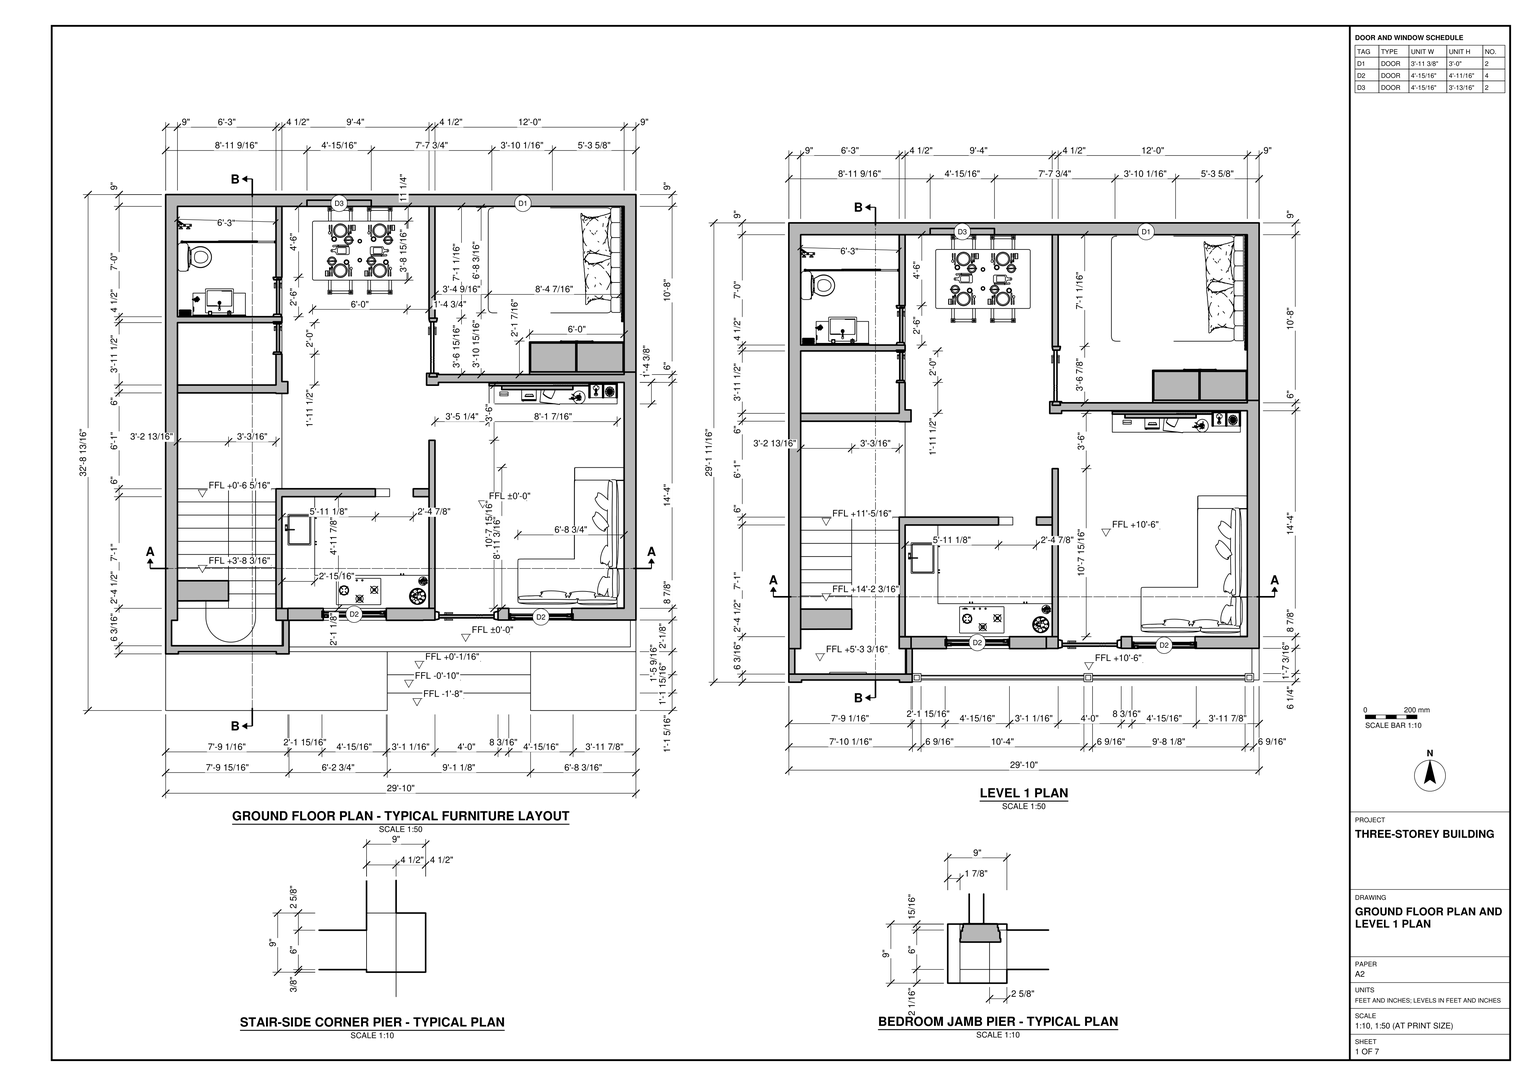
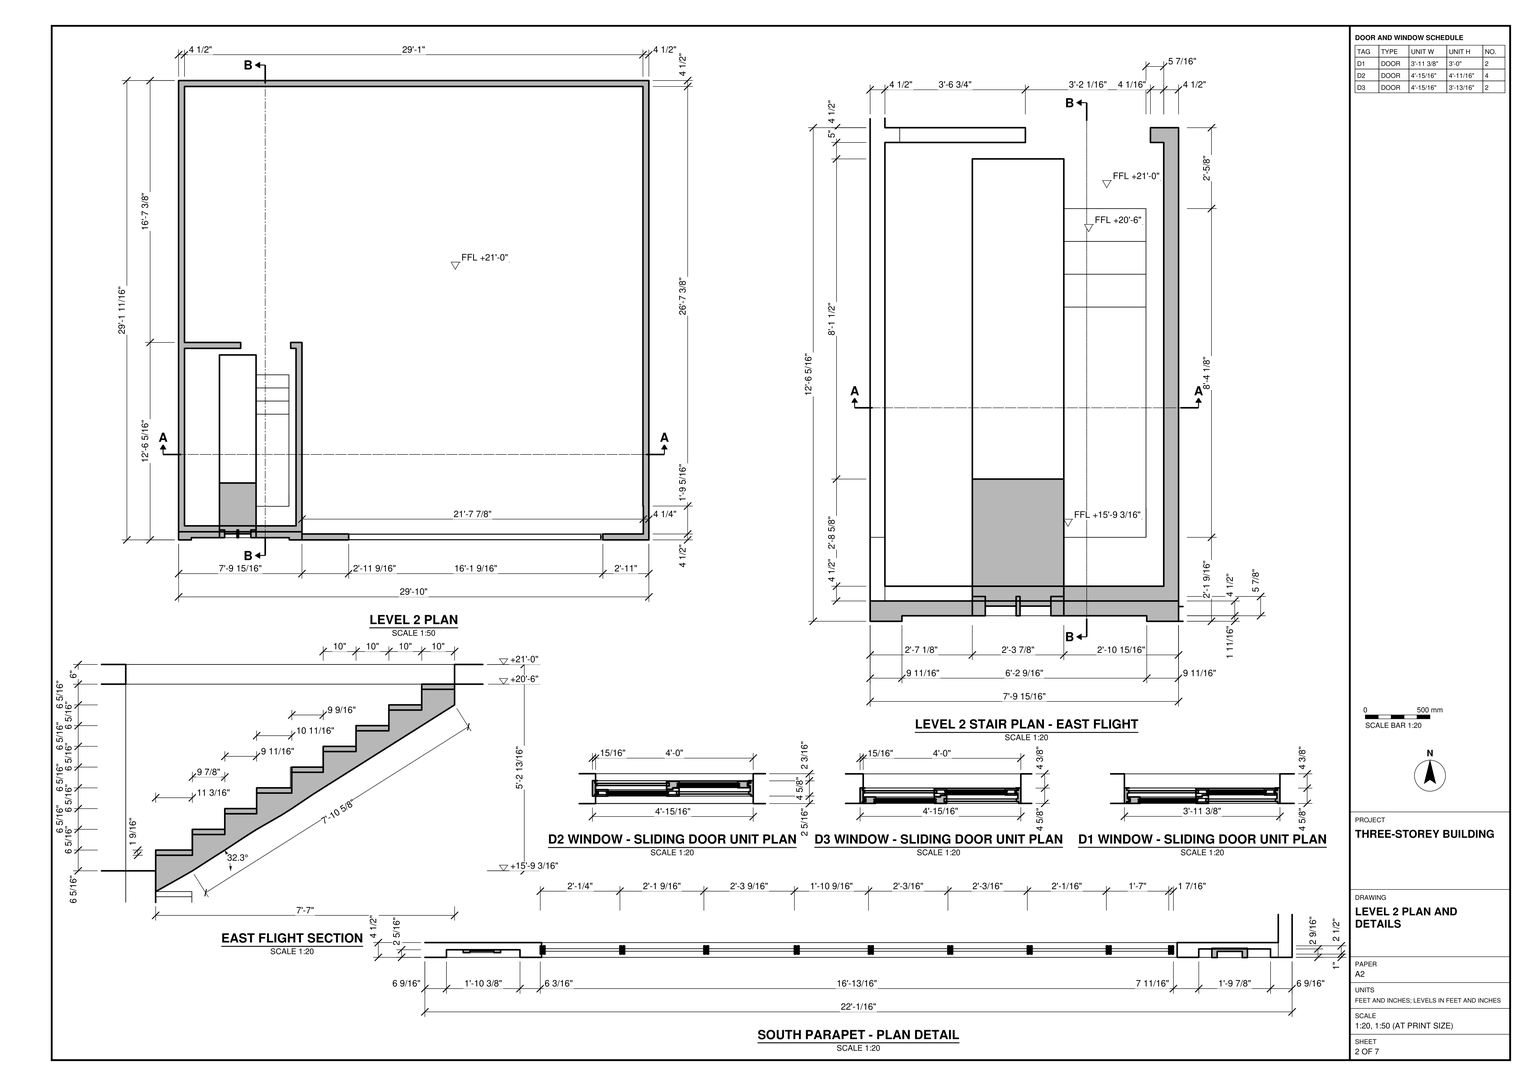
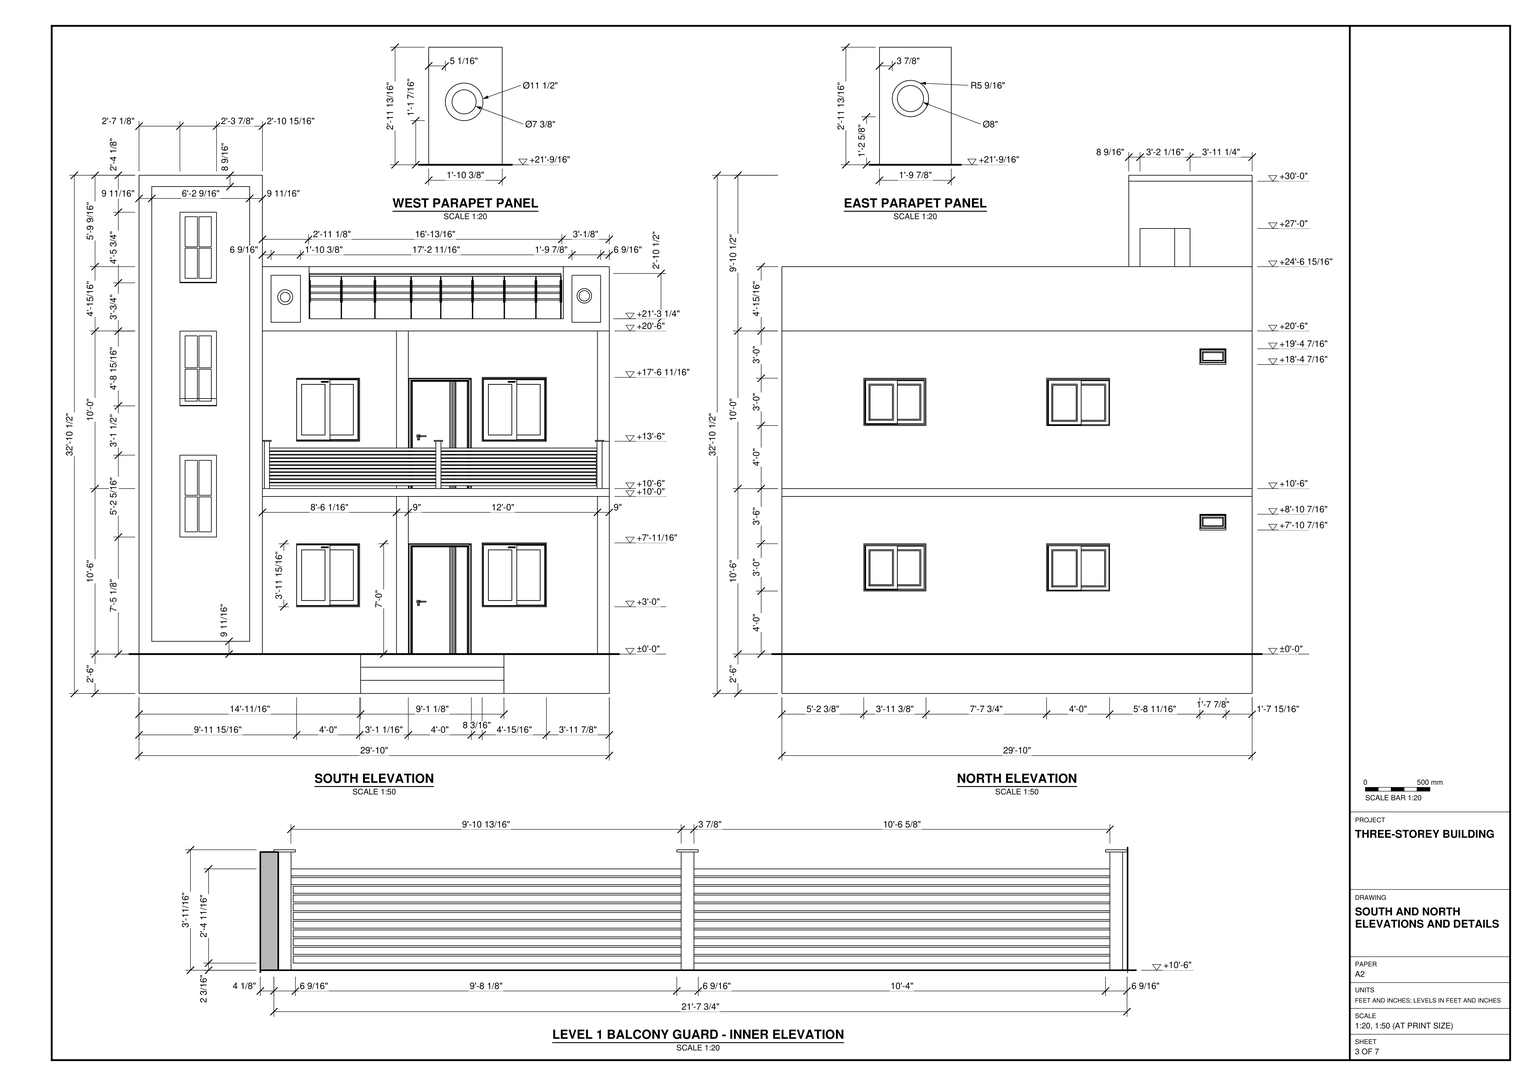
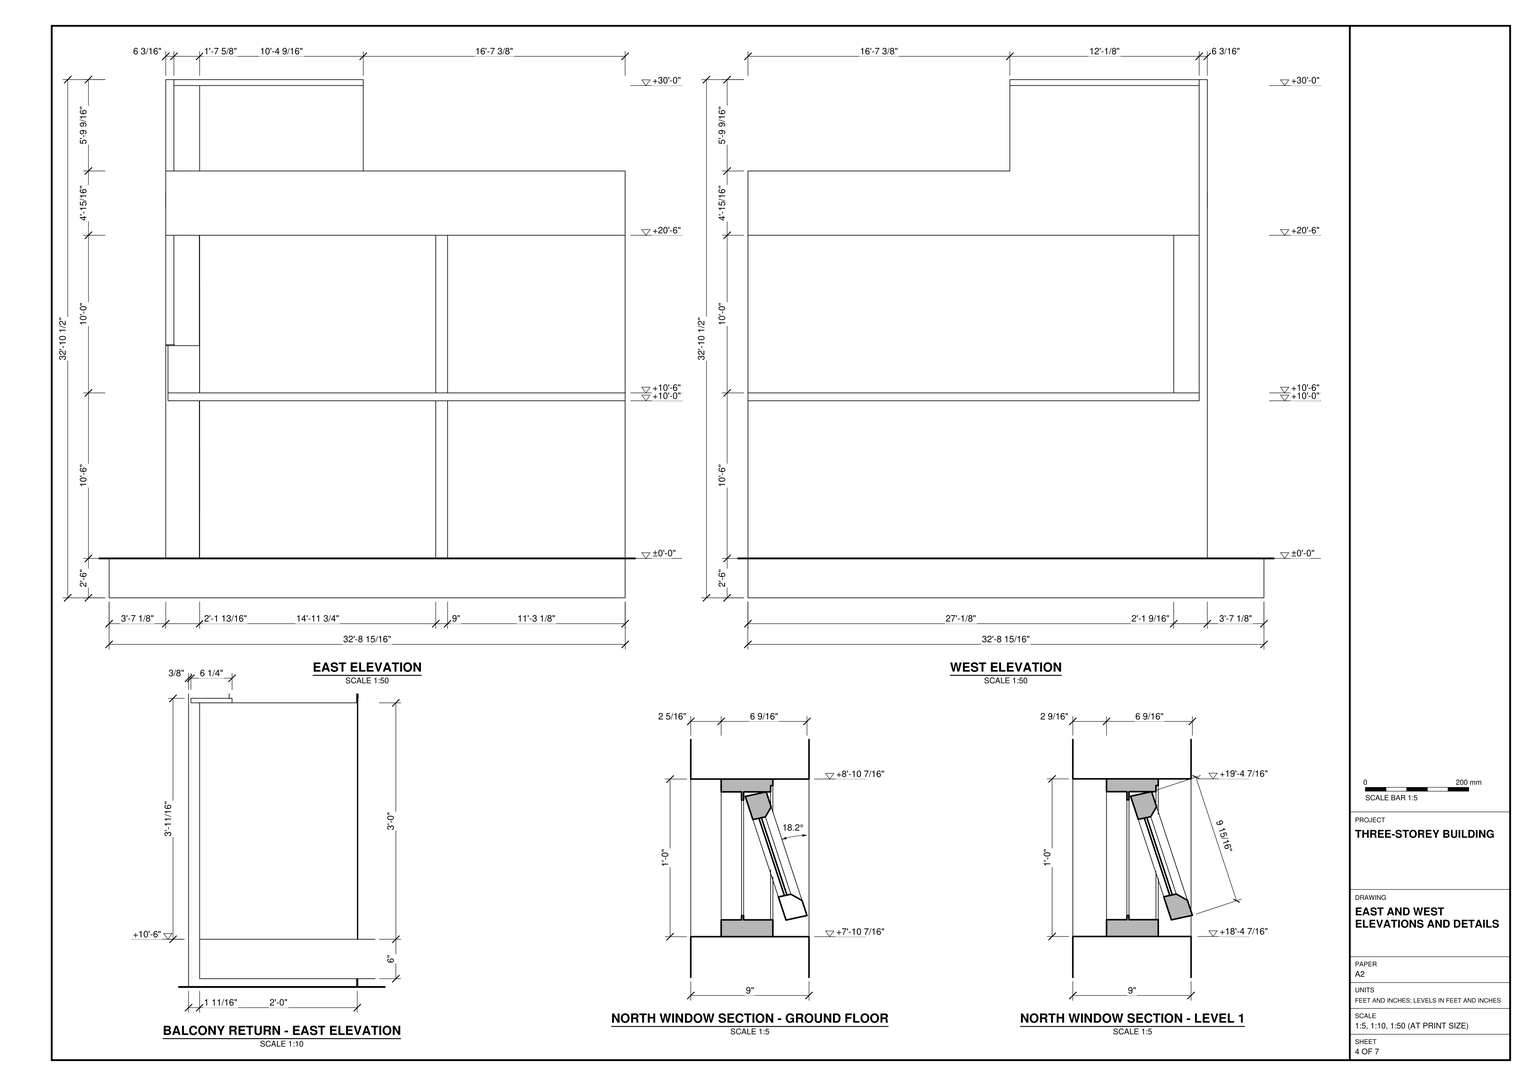
Build the residential building in SketchUp from task_files/diagram_01.pdf. Work in feet and inches. Orient the entrance toward the south and set the overall extents to 29'-10" east to west, 32'-8 15/16" north to south and 32'-10 1/2" from the base to the highest point. Use storey reference levels of ±0'-0", +10'-6" and +20'-6". Distinguish the upper reference level from the terrace surface at +21'-0".

Follow the ground-floor and Level 1 plans for the walls, piers, doorways and window openings. Use the wall thicknesses dimensioned at each location. On both furnished floors, place the stair at the southwest, the bathroom at the northwest, the dining area between the bathroom and bedroom, and the living area at the southeast. Fit the kitchen counters, sink and cooktop, and match the plan footprints and orientations of the dining table and chairs, bed, bedroom storage and corner sofa.

Model the base, entrance steps, floor slabs, stair flights and landings. Use the sections to carry the stair through to its enclosure above the flat roof terrace. Match the south elevation's stacked stair windows, Level 1 balcony guard and roof parapet with its rail opening and end panels.

Keep the walls, slabs and roof as separate groups or components, group each furniture or joinery piece separately, and use components for repeated parts. Decor and loose items may be any suitable library components. Save one SketchUp model as output_files/three_storey_residential_building_with_a_roof_terrace.skp.

# SketchUp Ruby script. Lengths in inches.
U = 1.inch
M = Sketchup.active_model
def pt(a) = Geom::Point3d.new(a.map { |v| v * U })
def face(e, loops, mat)
  f = e.add_face(loops[0].map { |a| pt(a) })
  loops[1..].each { |l| e.add_face(l.map { |a| pt(a) }).erase! }
  f.material = f.back_material = mat if mat
  f
end
# faces: each face lists its corners as indices into pts; further lists are holes
def faces(e, pts, list, mat = nil) = list.each { |f| face(e, (f[0].is_a?(Array) ? f : [f]).map { |l| l.map { |i| pts[i] } }, mat) }
# xy, xz, yz: faces in a plane at the given z, y or x. An outline is a flat list of corners, or four numbers for a rectangle; further outlines are holes
def ring(l) = l.size == 4 ? [[l[0], l[1]], [l[2], l[1]], [l[2], l[3]], [l[0], l[3]]] : l.each_slice(2).to_a
def flat(e, list, mat, &to3) = list.each { |f| face(e, (f[0].is_a?(Array) ? f : [f]).map { |l| ring(l).map { |u, v| to3.(u, v) } }, mat) }
def xy(e, z, list, mat = nil) = flat(e, list, mat) { |x, y| [x, y, z] }
def xz(e, y, list, mat = nil) = flat(e, list, mat) { |x, z| [x, y, z] }
def yz(e, x, list, mat = nil) = flat(e, list, mat) { |y, z| [x, y, z] }
def lines(e, pts, list) = list.each { |a, b| e.add_line(pt(pts[a]), pt(pts[b])) }
# prism: a flat outline (further loops are holes) pulled along v
def prism(e, loops, v, mat = nil)
  f = face(e, loops, mat); d = Geom::Vector3d.new(v.map { |x| x * U })
  f.pushpull(f.normal.samedirection?(d) ? d.length : -d.length)
end
def box(e, o, s, mat = nil) = prism(e, [[o, [o[0] + s[0], o[1], o[2]], [o[0] + s[0], o[1] + s[1], o[2]], [o[0], o[1] + s[1], o[2]]]], [0, 0, s[2]], mat)
def at(x, y, z, deg = 0) = Geom::Transformation.translation(pt([x, y, z])) * Geom::Transformation.rotation(ORIGIN, Z_AXIS, deg.degrees)
def axes(o, x, y, z) = Geom::Transformation.new([*x, 0, *y, 0, *z, 0, *pt(o).to_a, 1])
def part(name) = M.definitions.add(name)
# library, detail: a bought-in or finely detailed component or shape, given as its bounding box
def library(name, o, s) = part(name).tap { |d| box(d.entities, o, s) }
def detail(e, o, s) = box(e.add_group.entities, o, s)
def put(e, d, t, mat = nil) = e.add_instance(d, t).tap { |i| i.material = mat if mat }
def group(e, t, mat = nil) = e.add_group.tap { |g| g.transformation = t; g.material = mat if mat }.entities
root = M.entities
M.materials.add("[0042_Sienna]").color = [160, 82, 45]
M.materials.add("[0057_DarkKhaki]").color = [189, 183, 107]
M.materials.add("[0079_Teal]").color = [0, 128, 128]
M.materials.add("[0119_RosyBrown]").color = [188, 143, 143]
M.materials.add("[0123_DarkMagenta]").color = [139, 0, 139]
M.materials.add("[Basic Tile]").color = [203, 206, 202]
M.materials.add("[Carrera Marble]").color = [207, 207, 207]
M.materials.add("[Concrete Tile]").color = [203, 190, 164]
M.materials.add("[Granite Brown]").color = [126, 104, 91]
M.materials.add("[Granite Light Gray]").color = [149, 148, 144]
M.materials.add("[Metal Rough]").color = [153, 157, 160]
M.materials.add("[Stone Marble]").color = [143, 138, 136]
M.materials.add("[Wood Cherry Original]").color = [152, 86, 42]
M.materials.add("[Wood Veneer 01]").color = [120, 70, 37]
M.materials.add("brinjal velvet").color = [40, 45, 58]
c1 = part("Capped post")
xy(c1.entities,0,[[0,0,3.89,3.61]],"[0123_DarkMagenta]")
xy(c1.entities,36,[[[-1.33,-1.33,5.22,4.9375],[0,0,3.89,3.61]],[0,0,3.89,3.61]],"[0123_DarkMagenta]")
xy(c1.entities,36.6875,[[[-1.33,-1.33,5.22,4.9375],[0,0,3.89,3.61]]],"[0123_DarkMagenta]")
xz(c1.entities,-1.33,[[-1.33,36,5.22,36.6875]],"[0123_DarkMagenta]")
xz(c1.entities,0,[[0,0,3.89,36],[0,36,3.89,36.6875]],"[0123_DarkMagenta]")
xz(c1.entities,3.61,[[0,0,3.89,36],[0,36,3.89,36.6875]],"[0123_DarkMagenta]")
xz(c1.entities,4.9375,[[-1.33,36,5.22,36.6875]],"[0123_DarkMagenta]")
yz(c1.entities,-1.33,[[-1.33,36,4.9375,36.6875]],"[0123_DarkMagenta]")
yz(c1.entities,0,[[0,0,3.61,36],[0,36,3.61,36.6875]],"[0123_DarkMagenta]")
yz(c1.entities,3.89,[[0,0,3.61,36],[0,36,3.61,36.6875]],"[0123_DarkMagenta]")
yz(c1.entities,5.22,[[-1.33,36,4.9375,36.6875]],"[0123_DarkMagenta]")
c2 = library("Group\#141",[0,2.6,0],[24,6.53,12])
c3 = library("Group\#39",[0,0,0],[192.79,3.9375,24.79])
c4 = library("1-VASEFLEURS CLC2",[-4.93,-4.36,0],[9.88,8.02,19.93])
c5 = library("table dinner\#1",[0,0,0],[72,66.21,37.01])
c6 = part("WD_00_X1\#1")
p = [[-3.54,-3.54,0],[3.54,-3.54,0],[-3.54,3.54,0],[3.54,3.54,0],[3.39,0.71,0],[-3.39,0.71,0],
  [3.39,-0.71,0],[-3.39,-0.71,0],[-3.39,3.54,0],[-3.39,-3.54,0],[3.39,3.54,0],[3.39,-3.54,0]]
lines(c6.entities,p,[[0,1],[2,3],[4,5],[6,7],[8,9],[10,11]])
c7 = library("AS-120-mm\#1",[0,0,0],[47.36,4.72,36])
c8 = library("7-TABLE DE CUISSON CLC2",[-16.93,-10.04,0.13],[33.86,20.08,1.97])
c9 = library("My Toilet",[37.42,56.99,0],[19.17,25.6,30.6])
c10 = library("5-EVIER M60 CLC2\#1",[-11.69,-8.74,-7.125],[23.38,19.49,21.3])
c11 = library("AS-120-mm\#2",[0,0,0],[48.95,4.72,48.66])
c12 = library("BED 3",[-244.73,-59.6875,196.6875],[91.01,69.4,39.64])
c13 = library("3-PNGFRUITS CLC2",[-6.29,-6.27,0],[12.57,12.48,7.4])
c14 = library("tv unit model",[-7.7,0,0],[29.4,107.72,88.39])
c15 = library("AS-120-mm",[0,0,0],[48.95,4.72,36.79])
c16 = library("Photo frame",[10.08,0,11.14],[60,1.1,30])
c17 = library("skp5522",[0,-19.25,0],[30.73,19.25,144.92])
c18 = library("Group\#8",[0,-28.37,0],[77.61,119.5,120])
c19 = part("Group\#13")
prism(c19.entities,[[[4.5,0,0],[4.5,127.91,0],[4.5,127.91,84],[4.5,169.91,84],[4.5,169.91,120],[4.5,0,120]]],[-4.5,0,0])
c20 = part("Group\#11")
box(c20.entities,[0,0,0],[9,9,120])
c21 = part("Group\#14")
xy(c21.entities,0,[[0,0,102.97,9.11],[102.97,0.12,111.97,9.11]])
xy(c21.entities,36,[[26.9,0,74.9,9.11]])
xy(c21.entities,84,[[26.9,0,74.9,9.11]])
xy(c21.entities,120,[[0,0,102.97,0,102.97,0.12,111.97,0.12,111.97,9.11,0,9.11]])
xz(c21.entities,0,[[[0,0,102.97,120],[26.9,36,74.9,84]]])
xz(c21.entities,0.12,[[102.97,0,111.97,120]])
xz(c21.entities,9.11,[[[0,0,111.97,120],[26.9,36,74.9,84]]])
yz(c21.entities,0,[[0,0,9.11,120]])
yz(c21.entities,26.9,[[0,36,9.11,84]])
yz(c21.entities,74.9,[[0,36,9.11,84]])
yz(c21.entities,102.97,[[0,0,0.12,120]])
yz(c21.entities,111.97,[[0.12,0,9.11,120]])
c22 = part("Vertical batten")
box(c22.entities,[-1,0,-47.8125],[1,1.5625,96],"[0042_Sienna]")
c23 = part("Group\#178")
put(c23.entities,c22,at(1,81.15,47.8125))
put(c23.entities,c22,at(1,59.02,47.8125))
put(c23.entities,c22,at(1,46.73,47.8125))
put(c23.entities,c22,at(1,78.7,47.8125))
put(c23.entities,c22,at(1,68.86,47.8125))
put(c23.entities,c22,at(1,71.32,47.8125))
put(c23.entities,c22,at(1,66.4,47.8125))
put(c23.entities,c22,at(1,73.78,47.8125))
put(c23.entities,c22,at(1,63.94,47.8125))
put(c23.entities,c22,at(1,61.48,47.8125))
put(c23.entities,c22,at(1,56.5625,47.8125))
put(c23.entities,c22,at(1,76.24,47.8125))
put(c23.entities,c22,at(1,54.1,47.8125))
put(c23.entities,c22,at(1,49.18,47.8125))
put(c23.entities,c22,at(1,51.64,47.8125))
put(c23.entities,c22,at(1,24.59,47.8125))
put(c23.entities,c22,at(1,44.27,47.8125))
put(c23.entities,c22,at(1,41.81,47.8125))
put(c23.entities,c22,at(1,36.89,47.8125))
put(c23.entities,c22,at(1,29.51,47.8125))
put(c23.entities,c22,at(1,34.43,47.8125))
put(c23.entities,c22,at(1,31.97,47.8125))
put(c23.entities,c22,at(1,39.35,47.8125))
put(c23.entities,c22,at(1,27.05,47.8125))
put(c23.entities,c22,at(1,86.07,47.8125))
put(c23.entities,c22,at(1,9.84,47.8125))
put(c23.entities,c22,at(1,17.21,47.8125))
put(c23.entities,c22,at(1,12.3,47.8125))
put(c23.entities,c22,at(1,22.13,47.8125))
put(c23.entities,c22,at(1,19.67,47.8125))
put(c23.entities,c22,at(1,14.76,47.8125))
put(c23.entities,c22,at(1,2.46,47.8125))
put(c23.entities,c22,at(1,4.92,47.8125))
put(c23.entities,c22,at(1,7.38,47.8125))
put(c23.entities,c22,at(1,0,47.8125),"[0042_Sienna]")
put(c23.entities,c22,at(1,83.61,47.8125))
c24 = library("Group\#150",[0,0,0],[38.24,6.64,85.07])
c25 = library("Group\#21",[0,0,0],[6.64,44.74,84])
c26 = library("Group\#147",[0,0,0],[22.17,4.64,30.66])
c27 = library("Group\#149",[0,0,0],[72.18,1.14,83.07])
c28 = library("Group\#58",[0,-0.87,11.61],[44.14,21.23,59.64])
c29 = part("Group\#168")
xy(c29.entities,0,[[0,0,72,24]],"[Metal Rough]")
xy(c29.entities,0.75,[[0.75,2,71.25,24]],"[Metal Rough]")
xy(c29.entities,83.25,[[0.75,2,71.25,24]],"[Metal Rough]")
xy(c29.entities,84,[[0,0,72,24]],"[Metal Rough]")
xz(c29.entities,0,[[0,0,72,84]],"[Metal Rough]")
xz(c29.entities,2,[[0.75,0.75,71.25,83.25]],"[Metal Rough]")
xz(c29.entities,24,[[[0,0,72,84],[0.75,0.75,71.25,83.25]]],"[Metal Rough]")
yz(c29.entities,0,[[0,0,24,84]],"[Metal Rough]")
yz(c29.entities,0.75,[[2,0.75,24,83.25]],"[Metal Rough]")
yz(c29.entities,72,[[0,0,1.85,84],[1.85,0,24,84]],"[Metal Rough]")
g1 = group(c29.entities,at(71.25,2,0.75))
box(g1,[0,0,0],[0.75,22,82.5])
c30 = part("Group\#161")
prism(c30.entities,[[[72,1.85,0],[72,0,0],[0,0,0],[0,21,0],[72,21,0]]],[0,0,4],"[Metal Rough]")
c31 = library("Group\#172",[0,0,0],[72,1.4375,84])
c32 = library("Union\#1",[0,0,0],[70.5,22,82.5])
c33 = library("Group\#2",[0,0,0],[31.625,48.13,24])
c34 = library("Group\#26",[0,0,0],[29.625,48.13,24])
c35 = part("Group\#48")
xy(c35.entities,0,[[0,0,0,85,24.21,85,24.21,24.36,112,24.36,112,0]],"[Wood Veneer 01]")
xy(c35.entities,0.75,[[24.96,2.36,111.25,24.36],[2.21,25.11,24.21,84.25]],"[Wood Veneer 01]")
xy(c35.entities,29.25,[[24.96,2.36,111.25,24.36]],"[Wood Veneer 01]")
xz(c35.entities,0,[[0,0,112,30]],"[Wood Veneer 01]")
xz(c35.entities,2.36,[[24.96,0.75,111.25,29.25]],"[Wood Veneer 01]")
xz(c35.entities,24.36,[[[24.21,0,112,30],[24.96,0.75,111.25,29.25]]],"[Wood Veneer 01]")
xz(c35.entities,25.11,[[2.21,0.75,24.21,29.25]],"[Wood Veneer 01]")
xz(c35.entities,84.25,[[2.21,0.75,24.21,29.25]],"[Wood Veneer 01]")
xz(c35.entities,85,[[0,0,24.21,30]],"[Wood Veneer 01]")
yz(c35.entities,0,[[0,0,85,30]],"[Wood Veneer 01]")
yz(c35.entities,2.21,[[25.11,0.75,84.25,29.25]],"[Wood Veneer 01]")
yz(c35.entities,24.21,[[[24.36,0,85,30],[25.11,0.75,84.25,29.25]]],"[Wood Veneer 01]")
yz(c35.entities,24.96,[[2.36,0.75,24.36,29.25]],"[Wood Veneer 01]")
yz(c35.entities,111.25,[[2.36,0.75,24.36,29.25]],"[Wood Veneer 01]")
yz(c35.entities,112,[[0,0,24.36,30]],"[Wood Veneer 01]")
c36 = library("Group\#30",[0,0,0],[112,48.13,25.84])
c37 = library("Group\#38",[-7.59,0.01,0],[88.4,142.37,29.69])
c38 = library("Union",[0,0,0],[116.5,91,120])
c39 = library("Group\#51",[0,0,-18.1875],[112,85,20.1875])
c40 = library("Group\#29",[0,0,0],[87.79,60.64,30])
c41 = library("5-EVIER M60 CLC2",[-11.69,-8.74,-7.125],[23.38,19.49,21.3])
c42 = library("Group\#12",[0,0,0],[75.86,73.98,83.07])
c43 = library("Group773\#1",[-13.93,-31.17,0],[27.86,62.34,5.875])
c44 = library("Group775\#1",[-13.93,-31.11,0],[27.86,62.22,5.875])
c45 = library("Group\#45",[0,0,0],[126.65,2.125,28.6875])
c46 = library("Group\#36",[0,0,0],[118.84,2.125,28.6875])
c47 = library("Group\#162",[0,0,0],[11.12,2.8125,11.12])
c48 = library("Group\#146",[0,0,0],[11.44,0.875,11.44])
g2 = group(root,at(-123.84,0,-30))
g3 = group(g2,at(0,0,0))
xz(g3,68.69,[[169.22,276,207.84,282]],"[0119_RosyBrown]")
# 5 loose lines left out
put(g3,c1,at(219.26,44.8125,156))
put(g3,c1,at(349.8,44.8125,156))
put(g3,c1,at(472.48,44.8125,156))
put(g3,c2,axes([143.78,383.78,250.4375],[0.82813,0,0],[0,1,0],[0,0,1]))
put(g3,c3,axes([252.91,43.41,285.26],[1,0,0],[0,1,0],[0,0,1.3908]))
put(g3,c2,axes([143.78,383.53,124.4375],[0.82813,0,0],[0,1,0],[0,0,1]))
g4 = group(g3,at(123.84,49.3125,276),"[0119_RosyBrown]")
xy(g4,0,[[[93.91,-6.1875,358,-6.1875,358,343.5,0,343.5,0,0,93.91,0],[45.375,19.38,84,119.5]]])
xy(g4,6,[[[93.91,-1.6875,353.78,-1.6875,353.78,19.6,353.5,19.6,353.5,339,4.5,339,4.5,144.13,47.27,144.13,47.27,139.63,4.5,139.63,4.5,4.5,89.41,4.5,89.41,139.63,85.35,139.63,85.35,144.13,93.91,144.13],[45.375,19.38,84,119.5]]])
xy(g4,6.58,[[100.49,-6.1875,122.88,-3.875],[329.57,-6.1875,351.42,-3.625]])
xy(g4,9.26,[[129.46,-6.1875,322.99,-1.6875]])
xy(g4,37.07,[[31.12,0,58.98,37.125]])
xy(g4,42.37,[[100.49,-6.1875,122.88,-3.875],[329.57,-6.1875,351.42,-3.625]])
xy(g4,48.95,[[353.78,-6.1875,358,-6.1875,358,343.5,0,343.5,0,144.13,4.5,144.13,4.5,339,353.5,339,353.5,19.6,353.78,19.6],[93.91,-6.1875,129.46,-1.6875],[322.99,-6.1875,353.78,-1.6875]])
xy(g4,78,[[47.27,139.63,85.35,144.13]])
xy(g4,90.38,[[31.12,0,58.98,37.125]])
xy(g4,114,[[[0,0,93.91,144.13],[4.5,4.5,89.41,139.63]]])
xz(g4,-6.1875,[[[93.91,0,358,0,358,48.95,322.99,48.95,322.99,9.26,129.46,9.26,129.46,48.95,93.91,48.95],[100.49,6.58,122.88,42.37],[329.57,6.58,351.42,42.37]]])
xz(g4,-3.875,[[100.49,6.58,122.88,42.37]],"[0042_Sienna]")
xz(g4,-3.625,[[329.57,6.58,351.42,42.37]],"[0042_Sienna]")
xz(g4,-1.6875,[[93.91,6,129.46,48.95],[129.46,6,322.99,9.26],[322.99,6,353.78,48.95]])
xz(g4,0,[[[0,0,93.91,114],[31.12,37.07,58.98,90.38]]])
xz(g4,4.5,[[4.5,6,89.41,114]])
xz(g4,19.6,[[353.5,6,353.78,48.95]])
xz(g4,37.125,[[31.12,37.07,58.98,90.38]])
xz(g4,119.5,[[45.375,0,84,6]])
xz(g4,139.63,[[4.5,6,47.27,6,47.27,78,85.35,78,85.35,6,89.41,6,89.41,114,4.5,114]])
xz(g4,144.13,[[4.5,6,4.5,48.95,0,48.95,0,114,93.91,114,93.91,6,85.35,6,85.35,78,47.27,78,47.27,6]])
xz(g4,339,[[4.5,6,353.5,48.95]])
xz(g4,343.5,[[0,0,358,48.95]])
yz(g4,0,[[0,0,0,114,144.13,114,144.13,48.95,343.5,48.95,343.5,0]])
yz(g4,4.5,[[4.5,6,139.63,114],[144.13,6,339,48.95]])
yz(g4,31.12,[[0,37.07,37.125,90.38]])
yz(g4,45.375,[[19.38,0,119.5,6]])
yz(g4,47.27,[[139.63,6,144.13,78]])
yz(g4,58.98,[[0,37.07,37.125,90.38]])
yz(g4,84,[[19.38,0,119.5,6]])
yz(g4,85.35,[[139.63,6,144.13,78]])
yz(g4,89.41,[[4.5,6,19.38,114],[19.38,6,139.63,114]])
yz(g4,93.91,[[-6.1875,0,-6.1875,48.95,-1.6875,48.95,-1.6875,6,0,6,0,0],[0,6,19.6,114],[19.6,6,144.13,114]])
yz(g4,100.49,[[-6.1875,6.58,-3.875,42.37]])
yz(g4,122.88,[[-6.1875,6.58,-3.875,42.37]])
yz(g4,129.46,[[-6.1875,9.26,-1.6875,48.95]])
yz(g4,322.99,[[-6.1875,9.26,-1.6875,48.95]])
yz(g4,329.57,[[-6.1875,6.58,-3.625,42.37]])
yz(g4,351.42,[[-6.1875,6.58,-3.625,42.37]])
yz(g4,353.5,[[19.6,6,339,48.95]])
yz(g4,353.78,[[-1.6875,6,19.6,48.95]])
yz(g4,358,[[-6.1875,0,343.5,48.95]])
# 6 loose lines left out
g5 = group(g3,at(476.37,44.8125,156),"[0079_Teal]")
box(g5,[0,0,0],[5.47,24,36])
g6 = group(g3,at(123.84,49.3125,390),"[0119_RosyBrown]")
box(g6,[0,0,0],[93.91,144.13,4.5])
g7 = group(g3,at(123.84,31.5,150))
xy(g7,6,[[261.2,37.41,349,46.3125],[349,37.41,358,46.3125],[349,46.3125,358,46.41],[349,46.41,358,217.16],[84,209.93,88.5,218.93],
  [88.5,209.93,93,218.93],[9,210.3125,84,216.3125],[198.64,216.22,200.5,225.22],[200.5,216.22,205,218.3125],[205,216.22,207.64,218.3125],
  [349,217.16,358,226.16],[200.5,218.3125,205,224.3125],[205,218.3125,207.64,224.3125],[207.64,218.3125,349,224.3125],[84,218.93,88.5,239.8125],
  [200.5,224.3125,205,225.22],[205,224.3125,207.64,225.22],[200.5,267.22,205,352.3125]])
xy(g7,6,[[0,37.1875,4.5,46.1875],[84.03,37.19,88.5,37.3125],[88.5,37.19,89.41,37.3125],[89.41,37.19,93.03,37.3125],[84.03,37.3125,88.5,46.19],
  [88.5,37.3125,93.03,46.19],[349,226.16,358,352.3125],[84,298.3125,88.5,352.29],[84,352.29,88.5,352.3125],[0,352.3125,9,361.3125],
  [9,352.3125,81.16,352.3125,81.16,361.29,90.16,361.29,90.16,361.3125,9,361.3125],[81.16,352.3125,90.16,361.29],[90.16,352.3125,349,352.3125,349,361.3125,206.63,361.3125,206.63,352.4,197.63,352.4,197.63,361.3125,90.16,361.3125],[197.63,352.4,206.63,361.3125]],"[0057_DarkKhaki]")
xy(g7,42,[[261.2,37.41,309.2,46.3125]],"[0057_DarkKhaki]")
xy(g7,54,[[108.52,352.3125,156.52,361.3125],[248.29,352.3125,295.65,361.3125]],"[0057_DarkKhaki]")
xy(g7,90,[[205,37.41,253,46.3125],[261.2,37.41,309.2,46.3125],[200.5,225.22,205,267.22]])
xy(g7,90,[[84,239.8125,88.5,263.8125],[84,268.3125,88.5,298.3125],[108.52,352.3125,156.52,361.3125],[248.29,352.3125,295.65,361.3125]],"[0057_DarkKhaki]")
xy(g7,100.4375,[[19.9375,352.3125,39.8125,361.3125]],"[0057_DarkKhaki]")
xy(g7,112.4375,[[19.9375,352.3125,39.8125,361.3125]],"[0057_DarkKhaki]")
xy(g7,126,[[0,37.1875,9,208.85],[205,37.41,358,37.41,358,217.16,349,217.16,349,46.3125,205,46.3125],[0,208.85,9,208.85,9,263.8125,88.5,263.8125,88.5,352.29,84,352.29,84,268.3125,9,268.3125,9,352.3125,349,352.3125,349,226.16,358,226.16,358,361.3125,0,361.3125],[84,209.93,93,209.93,93,218.93,88.5,218.93,88.5,263.8125,84,263.8125,84,216.3125,9,216.3125,9,210.3125,84,210.3125],[198.64,216.22,207.64,216.22,207.64,218.3125,349,218.3125,349,217.16,358,217.16,358,226.16,349,226.16,349,224.3125,207.64,224.3125,207.64,225.22,205,225.22,205,352.3125,200.5,352.3125,200.5,225.22,198.64,225.22]],"[0057_DarkKhaki]")
xz(g7,17.8125,[[88.5,6,89.41,126]],"[0057_DarkKhaki]")
xz(g7,37.1875,[[0,6,4.5,126],[4.5,6,9,126]],"[0057_DarkKhaki]")
xz(g7,37.19,[[89.41,6,93.03,126],[93.03,6,93.91,126]],"[0057_DarkKhaki]")
xz(g7,37.41,[[[253,6,349,6,349,126,205,126,205,90,253,90],[261.2,42,309.2,90]],[349,6,358,126]],"[0057_DarkKhaki]")
xz(g7,46.3125,[[[253,6,253,90,205,90,205,126,349,126,349,6],[261.2,42,309.2,90]]],"[0057_DarkKhaki]")
xz(g7,209.93,[[84,6,93,126]],"[0057_DarkKhaki]")
xz(g7,210.3125,[[9,6,84,126]],"[0057_DarkKhaki]")
xz(g7,216.22,[[198.64,6,207.64,126]],"[0057_DarkKhaki]")
xz(g7,216.3125,[[9,6,84,126]],"[0057_DarkKhaki]")
xz(g7,218.3125,[[207.64,6,349,126]],"[0057_DarkKhaki]")
xz(g7,218.93,[[88.5,6,93,126]],"[0057_DarkKhaki]")
xz(g7,224.3125,[[207.64,6,349,126]],"[0057_DarkKhaki]")
xz(g7,225.22,[[198.64,6,198.64,126,200.5,126,200.5,90,205,90,205,126,207.64,126,207.64,6]],"[0057_DarkKhaki]")
xz(g7,226.16,[[349,6,358,126]],"[0057_DarkKhaki]")
xz(g7,239.8125,[[84,6,88.5,90]],"[0057_DarkKhaki]")
xz(g7,263.8125,[[9,6,88.5,6,88.5,90,84,90,84,126,9,126],[84,90,88.5,126]],"[0057_DarkKhaki]")
xz(g7,267.22,[[200.5,6,205,90]])
xz(g7,268.3125,[[9,6,9,126,84,126,84,90,88.5,90,88.5,6]],"[Granite Light Gray]")
xz(g7,298.3125,[[84,6,88.5,90]],"[0057_DarkKhaki]")
xz(g7,352.29,[[84,6,88.5,126]],"[0057_DarkKhaki]")
xz(g7,352.3125,[[200.5,6,205,126]])
xz(g7,352.3125,[[[9,6,200.5,126],[108.52,54,156.52,90],[19.9375,100.4375,39.8125,112.4375]],[[205,6,349,126],[248.29,54,295.65,90]]],"[0057_DarkKhaki]")
xz(g7,361.3125,[[[0,6,358,126],[108.52,54,156.52,90],[248.29,54,295.65,90],[19.9375,100.4375,39.8125,112.4375]]],"[0057_DarkKhaki]")
yz(g7,0,[[37.1875,6,361.3125,126]],"[0057_DarkKhaki]")
yz(g7,9,[[210.3125,6,216.3125,126]])
yz(g7,9,[[37.1875,6,208.85,126],[208.85,6,210.3125,126],[216.3125,6,217.85,126],[217.85,6,263.8125,126]],"[0057_DarkKhaki]")
yz(g7,9,[[268.3125,6,352.3125,126]],"[Granite Light Gray]")
yz(g7,19.9375,[[352.3125,100.4375,361.3125,112.4375]],"[0057_DarkKhaki]")
yz(g7,39.8125,[[352.3125,100.4375,361.3125,112.4375]],"[0057_DarkKhaki]")
yz(g7,84,[[209.93,6,210.3125,126],[216.3125,6,218.93,126],[218.93,6,218.93,126,263.8125,126,263.8125,90,239.8125,90,239.8125,6]],"[0057_DarkKhaki]")
yz(g7,84,[[298.3125,6,298.3125,90,268.3125,90,268.3125,126,352.29,126,352.29,6]],"[Granite Light Gray]")
yz(g7,88.5,[[218.93,6,239.8125,6,239.8125,90,263.8125,90,263.8125,126,218.93,126],[263.8125,6,268.3125,6,268.3125,90,298.3125,90,298.3125,6,352.29,6,352.29,126,263.8125,126]],"[0057_DarkKhaki]")
yz(g7,89.41,[[17.8125,6,37.19,126]],"[0057_DarkKhaki]")
yz(g7,93,[[209.93,6,218.93,126]],"[0057_DarkKhaki]")
yz(g7,108.52,[[352.3125,54,361.3125,90]],"[0057_DarkKhaki]")
yz(g7,156.52,[[352.3125,54,361.3125,90]],"[0057_DarkKhaki]")
yz(g7,198.64,[[216.22,6,225.22,126]],"[0057_DarkKhaki]")
yz(g7,200.5,[[267.22,6,267.22,90,225.22,90,225.22,126,352.3125,126,352.3125,6]],"[0057_DarkKhaki]")
yz(g7,205,[[37.41,90,46.3125,126]])
yz(g7,205,[[267.22,6,352.3125,6,352.3125,126,225.22,126,225.22,90,267.22,90]],"[0057_DarkKhaki]")
yz(g7,207.64,[[216.22,6,218.3125,126],[224.3125,6,225.22,126]],"[0057_DarkKhaki]")
yz(g7,248.29,[[352.3125,54,361.3125,90]],"[0057_DarkKhaki]")
yz(g7,253,[[37.41,6,46.3125,90]])
yz(g7,261.2,[[37.41,42,46.3125,90]],"[0057_DarkKhaki]")
yz(g7,295.65,[[352.3125,54,361.3125,90]],"[0057_DarkKhaki]")
yz(g7,309.2,[[37.41,42,46.3125,90]],"[0057_DarkKhaki]")
yz(g7,349,[[217.16,6,218.3125,126],[224.3125,6,226.16,10]])
yz(g7,349,[[46.3125,6,217.16,126],[226.16,6,352.3125,126],[224.3125,10,226.16,126]],"[0057_DarkKhaki]")
yz(g7,358,[[37.41,6,217.16,126],[217.16,6,226.16,126],[226.16,6,361.3125,126]],"[0057_DarkKhaki]")
# 143 loose lines left out
put(g7,c4,at(195.84,67.02,38))
put(g7,c5,at(111.77,285.48,11.18))
put(g7,c6,axes([143.9375,41.75,6],[6.78823,0,0],[0,1.27279,0],[0,0,6.78823]))
put(g7,c7,at(248.29,352.3125,54))
put(g7,c8,axes([146.88,59.08,38],[1,0,0],[0,-1,0],[0,0,1]))
put(g7,c6,axes([132.52,356.8125,6],[-6.78823,0,0],[0,1.27279,0],[0,0,6.78823]))
put(g7,c9,axes([91.93,261.04,6.08],[0,1.12,0],[-1,0,0],[0,0,1.3013]))
put(g7,c10,at(101.8,106.13,38.07,90))
put(g7,c11,at(118.99,39.47,42))
put(g7,c12,axes([68.77,280.53,-191.07],[-1.15,0,0],[0,-1.27931,0],[0,0,1]))
put(g7,c6,axes([284.24,41.8125,6],[6.78823,0,0],[0,-1.27279,0],[0,0,6.78823]))
put(g7,c6,axes([21,356.8125,6],[3.39411,0,0],[0,1.27279,0],[0,0,3.39411]))
put(g7,c13,at(191.79,55.46,38))
put(g7,c11,at(261.2,37.41,42))
put(g7,c14,axes([246.23,201.5,22.14],[0,1,0],[0.9048,0,0],[0,0,1]))
put(g7,c6,axes([271.33,356.8125,6],[6.78823,0,0],[0,1.27279,0],[0,0,6.78823]))
put(g7,c15,at(107.57,352.3125,53.21))
put(g7,c16,axes([206.1,354.53,70.9],[0,-1,0],[-1,0,0],[0,0,1]))
put(g7,c17,axes([19.66,335.08,25.85],[-0.375,0,0],[0,-0.375,0],[0,0,0.375]))
put(g7,c18,at(9,46.1875,6),"[Carrera Marble]")
put(g7,c19,at(200.5,46.3125,6),"[0057_DarkKhaki]")
put(g7,c20,at(84.03,37.19,6),"[0057_DarkKhaki]")
put(g7,c21,at(93.03,37.19,6),"[0057_DarkKhaki]")
put(g7,c23,at(347.25,264.68,6))
put(g7,c24,axes([88.5,268.3125,6],[0,0.78451,0],[-1,0,0],[0,0,0.98748]))
put(g7,c25,at(200.06,222.48,6))
put(g7,c26,axes([20.79,273.25,35.96],[-0.5414,0,0],[0,-1,0],[0,0,1]))
put(g7,c27,at(11.82,324.67,5.21))
put(g7,c28,axes([60.7,288.68,18.45],[-0.91,0,0],[0,-1,0],[0,0,0.95]))
put(g7,c29,at(277,224.3125,10),"[Wood Cherry Original]")
put(g7,c24,axes([88.5,239.8125,6],[0,0.6433,0],[-1,0,0],[0,0,0.98748]))
put(g7,c30,at(277,224.3125,6),"[Stone Marble]")
put(g7,c25,axes([253,37.21,6.03],[0,1,0],[-1.07284,0,0],[0,0,1]))
put(g7,c31,at(277,248.3125,10))
put(g7,c32,at(277.75,226.3125,10.75))
put(g7,c33,at(88.5,46.3125,66))
put(g7,c34,axes([200.5,46.3125,65.91],[-1,0,0],[0,1,0],[0,0,1]))
put(g7,c35,at(88.5,46.3125,6))
put(g7,c36,at(88.5,46.3125,90.1))
put(g7,c37,axes([275.06,46.7,5.59],[0.91489,0,0],[0,0.7502,0],[0,0,1.63]),"brinjal velvet")
put(g7,c38,at(84,46.3125,6),"[0057_DarkKhaki]")
g8 = group(g7,at(0,13.3125,0))
p = [[9,23.875,6],[9,23.875,0],[93.91,4.5,0],[93.91,4.5,6]]
lines(g8,p,[[0,1],[2,3]])
put(g8,c39,at(88.5,33,36),"[Stone Marble]")
g9 = group(g8,at(0,24,0),"[Basic Tile]")
xy(g9,0,[[93.91,-24,93.91,-19.5,88.5,-19.5,88.5,-0.2,84,-0.2,84,100,9,100,9,-0.125,4.5,-0.125,4.5,-19.5,0,-19.5,0,324,358,324,358,-24]])
xy(g9,6,[[93.91,-24,358,-24,358,324,0,324,0,-0.125,9,-0.125,9,100,84,100,84,-0.2,88.5,-0.2,88.5,-19.5,93.91,-19.5],[0,-19.5,4.5,-0.125]],"[Concrete Tile]")
xz(g9,-24,[[93.91,0,358,6]])
xz(g9,-19.5,[[0,0,4.5,6],[88.5,0,93.91,6]])
xz(g9,-0.2,[[84,0,88.5,6]])
xz(g9,-0.125,[[4.5,0,9,6]])
xz(g9,100,[[9,0,84,6]])
xz(g9,324,[[0,0,358,6]])
yz(g9,0,[[-19.5,0,324,6]])
yz(g9,4.5,[[-19.5,0,-0.125,6]])
yz(g9,9,[[-0.125,0,100,6]])
yz(g9,84,[[-0.2,0,100,6]])
yz(g9,88.5,[[-19.5,0,-0.2,6]])
yz(g9,93.91,[[-24,0,-19.5,6]])
yz(g9,358,[[-24,0,324,6]])
# 5 loose lines left out
put(g8,c40,at(112.71,57.36,6))
g10 = group(g7,at(0,13.3125,6),"[0057_DarkKhaki]")
box(g10,[0,4.5,0],[4.5,19.375,120])
xy(g10,0,[[89.35,4.5,93.91,23.88],[93.03,23.88,196,32.99]])
xy(g10,120,[[89.35,4.5,93.91,23.88],[84,23.88,196,23.88,196,32.99,93.03,32.99,93.03,33,84,33]])
xz(g10,4.5,[[89.35,0,93.91,120]])
xz(g10,23.88,[[84,0,89.35,120],[89.35,0,93.03,120],[93.03,0,93.91,120]])
xz(g10,32.99,[[[93.03,0,196,120],[119.9375,36,167.9375,84]]])
xz(g10,33,[[84,0,93.03,120]])
yz(g10,84,[[23.88,0,33,120]])
yz(g10,89.35,[[4.5,0,23.88,120]])
yz(g10,93.03,[[32.99,0,33,120]])
yz(g10,93.91,[[4.5,0,23.88,120]])
yz(g10,196,[[23.88,0,32.99,120]])
# 1 loose lines left out
g11 = group(g3,at(123.84,31.5,24))
xy(g11,6,[[261.2,37.41,349,46.3125],[349,37.41,358,46.3125],[349,46.3125,358,46.41],[349,46.41,358,217.16],[84,209.93,88.5,218.93],
  [88.5,209.93,93,218.93],[9,210.3125,84,216.3125],[198.64,216.22,200.5,225.22],[200.5,216.22,205,218.3125],[205,216.22,207.64,218.3125],
  [349,217.16,358,226.16],[200.5,218.3125,205,224.3125],[205,218.3125,207.64,224.3125],[207.64,218.3125,349,224.3125],[84,218.93,88.5,239.8125],
  [200.5,224.3125,205,225.22],[205,224.3125,207.64,225.22],[200.5,267.22,205,352.3125]])
xy(g11,6,[[0,11.625,0,37.1875,4.5,37.1875,4.5,17.8125,89.41,17.8125,89.41,37.19,93.91,37.19,93.91,11.625],[0,37.1875,4.5,46.1875],[84.03,37.19,88.5,37.3125],[88.5,37.19,89.41,37.3125],[89.41,37.19,93.03,37.3125],
  [84.03,37.3125,88.5,46.19],[88.5,37.3125,93.03,46.19],[349,226.16,358,352.3125],[84,298.3125,88.5,352.29],[84,352.29,88.5,352.3125],
  [0,352.3125,9,361.3125],[9,352.3125,81.16,352.3125,81.16,361.29,90.16,361.29,90.16,361.3125,9,361.3125],[81.16,352.3125,90.16,361.29],[90.16,352.3125,349,352.3125,349,361.3125,206.63,361.3125,206.63,352.4,197.63,352.4,197.63,361.3125,90.16,361.3125],[197.63,352.4,206.63,361.3125]],"[0057_DarkKhaki]")
xy(g11,15.68,[[9.68,11.625,84.23,13.3125]],"[0079_Teal]")
xy(g11,42,[[261.2,37.41,309.2,46.3125]],"[0057_DarkKhaki]")
xy(g11,54,[[108.52,352.3125,156.52,361.3125],[248.29,352.3125,295.65,361.3125]],"[0057_DarkKhaki]")
xy(g11,90,[[205,37.41,253,46.3125],[261.2,37.41,309.2,46.3125],[200.5,225.22,205,267.22]])
xy(g11,90,[[84,239.8125,88.5,263.8125],[84,268.3125,88.5,298.3125],[108.52,352.3125,156.52,361.3125],[248.29,352.3125,295.65,361.3125]],"[0057_DarkKhaki]")
xy(g11,95.1,[[31.12,13.3125,58.98,17.8125]],"[0079_Teal]")
xy(g11,100.4375,[[19.9375,352.3125,39.8125,361.3125]],"[0057_DarkKhaki]")
xy(g11,112.4375,[[19.9375,352.3125,39.8125,361.3125]],"[0057_DarkKhaki]")
xy(g11,126,[[0,17.8125,4.5,37.1875],[89.41,17.8125,93.91,37.19],[0,37.1875,9,208.85],[205,37.41,358,37.41,358,217.16,349,217.16,349,46.3125,205,46.3125],[0,208.85,9,208.85,9,263.8125,88.5,263.8125,88.5,352.29,84,352.29,84,268.3125,9,268.3125,9,352.3125,349,352.3125,349,226.16,358,226.16,358,361.3125,0,361.3125],
  [84,209.93,93,209.93,93,218.93,88.5,218.93,88.5,263.8125,84,263.8125,84,216.3125,9,216.3125,9,210.3125,84,210.3125],[198.64,216.22,207.64,216.22,207.64,218.3125,349,218.3125,349,217.16,358,217.16,358,226.16,349,226.16,349,224.3125,207.64,224.3125,207.64,225.22,205,225.22,205,352.3125,200.5,352.3125,200.5,225.22,198.64,225.22]],"[0057_DarkKhaki]")
xy(g11,157.43,[[31.12,13.3125,58.98,17.8125]],"[0079_Teal]")
xy(g11,195.34,[[31.12,13.3125,58.98,17.8125]],"[0079_Teal]")
xy(g11,251.88,[[31.12,13.3125,58.98,17.8125]],"[0079_Teal]")
xy(g11,289.07,[[31.12,13.3125,58.98,152.4375]],"[0079_Teal]")
xy(g11,342.38,[[31.12,13.3125,58.98,152.4375]],"[0079_Teal]")
xy(g11,361.94,[[9.68,11.625,84.23,13.3125]],"[0079_Teal]")
xy(g11,370.5,[[0,11.625,93.91,17.8125]],"[0057_DarkKhaki]")
xz(g11,11.625,[[[0,6,93.91,370.5],[9.68,15.68,84.23,361.94]]],"[0123_DarkMagenta]")
xz(g11,13.3125,[[[9.68,15.68,84.23,361.94],[31.12,95.1,58.98,157.43],[31.12,195.34,58.98,251.88],[31.12,289.07,58.98,342.38]]],"[0079_Teal]")
xz(g11,17.8125,[[[4.5,6,4.5,126,0,126,0,370.5,93.91,370.5,93.91,126,89.41,126,89.41,6],[31.12,95.1,58.98,157.43],[31.12,195.34,58.98,251.88]]],"[0057_DarkKhaki]")
xz(g11,37.1875,[[4.5,6,9,126]],"[0057_DarkKhaki]")
xz(g11,37.19,[[89.41,6,93.03,126],[93.03,6,93.91,126]],"[0057_DarkKhaki]")
xz(g11,37.41,[[[253,6,349,6,349,126,205,126,205,90,253,90],[261.2,42,309.2,90]],[349,6,358,126]],"[0057_DarkKhaki]")
xz(g11,46.3125,[[[253,6,253,90,205,90,205,126,349,126,349,6],[261.2,42,309.2,90]]],"[0057_DarkKhaki]")
xz(g11,152.4375,[[31.12,289.07,58.98,342.38]],"[0079_Teal]")
xz(g11,209.93,[[84,6,93,126]],"[0057_DarkKhaki]")
xz(g11,210.3125,[[9,6,84,126]],"[0057_DarkKhaki]")
xz(g11,216.22,[[198.64,6,207.64,126]],"[0057_DarkKhaki]")
xz(g11,216.3125,[[9,6,84,126]],"[0057_DarkKhaki]")
xz(g11,218.3125,[[207.64,6,349,126]],"[0057_DarkKhaki]")
xz(g11,218.93,[[88.5,6,93,126]],"[0057_DarkKhaki]")
xz(g11,224.3125,[[207.64,6,349,126]],"[0057_DarkKhaki]")
xz(g11,225.22,[[198.64,6,198.64,126,200.5,126,200.5,90,205,90,205,126,207.64,126,207.64,6]],"[0057_DarkKhaki]")
xz(g11,226.16,[[349,6,358,126]],"[0057_DarkKhaki]")
xz(g11,239.8125,[[84,6,88.5,90]],"[0057_DarkKhaki]")
xz(g11,263.8125,[[9,6,88.5,6,88.5,90,84,90,84,126,9,126],[84,90,88.5,126]],"[0057_DarkKhaki]")
xz(g11,267.22,[[200.5,6,205,90]])
xz(g11,268.3125,[[9,6,9,126,84,126,84,90,88.5,90,88.5,6]],"[Granite Light Gray]")
xz(g11,298.3125,[[84,6,88.5,90]],"[0057_DarkKhaki]")
xz(g11,352.29,[[84,6,88.5,126]],"[0057_DarkKhaki]")
xz(g11,352.3125,[[200.5,6,205,126]])
xz(g11,352.3125,[[[9,6,200.5,126],[108.52,54,156.52,90],[19.9375,100.4375,39.8125,112.4375]],[[205,6,349,126],[248.29,54,295.65,90]]],"[0057_DarkKhaki]")
xz(g11,361.3125,[[[0,6,358,126],[108.52,54,156.52,90],[248.29,54,295.65,90],[19.9375,100.4375,39.8125,112.4375]]],"[0057_DarkKhaki]")
yz(g11,0,[[11.625,6,11.625,370.5,17.8125,370.5,17.8125,126,361.3125,126,361.3125,6]],"[0057_DarkKhaki]")
yz(g11,4.5,[[17.8125,6,37.1875,126]],"[0057_DarkKhaki]")
yz(g11,9,[[210.3125,6,216.3125,126]])
yz(g11,9,[[37.1875,6,208.85,126],[208.85,6,210.3125,126],[216.3125,6,217.85,126],[217.85,6,263.8125,126]],"[0057_DarkKhaki]")
yz(g11,9,[[268.3125,6,352.3125,126]],"[Granite Light Gray]")
yz(g11,9.68,[[11.625,15.68,13.3125,361.94]],"[0079_Teal]")
yz(g11,19.9375,[[352.3125,100.4375,361.3125,112.4375]],"[0057_DarkKhaki]")
yz(g11,31.12,[[13.3125,95.1,17.8125,157.43],[13.3125,195.34,17.8125,251.88],[13.3125,289.07,152.4375,342.38]],"[0079_Teal]")
yz(g11,39.8125,[[352.3125,100.4375,361.3125,112.4375]],"[0057_DarkKhaki]")
yz(g11,58.98,[[13.3125,95.1,17.8125,157.43],[13.3125,195.34,17.8125,251.88],[13.3125,289.07,152.4375,342.38]],"[0079_Teal]")
yz(g11,84,[[209.93,6,210.3125,126],[216.3125,6,218.93,126],[218.93,6,218.93,126,263.8125,126,263.8125,90,239.8125,90,239.8125,6]],"[0057_DarkKhaki]")
yz(g11,84,[[298.3125,6,298.3125,90,268.3125,90,268.3125,126,352.29,126,352.29,6]],"[Granite Light Gray]")
yz(g11,84.23,[[11.625,15.68,13.3125,361.94]],"[0079_Teal]")
yz(g11,88.5,[[218.93,6,239.8125,6,239.8125,90,263.8125,90,263.8125,126,218.93,126],[263.8125,6,268.3125,6,268.3125,90,298.3125,90,298.3125,6,352.29,6,352.29,126,263.8125,126]],"[0057_DarkKhaki]")
yz(g11,89.41,[[17.8125,6,37.19,126]],"[0057_DarkKhaki]")
yz(g11,93,[[209.93,6,218.93,126]],"[0057_DarkKhaki]")
yz(g11,93.91,[[11.625,6,37.19,6,37.19,126,17.8125,126,17.8125,300.95,11.625,300.95],[11.625,300.95,17.8125,370.5]],"[0057_DarkKhaki]")
yz(g11,108.52,[[352.3125,54,361.3125,90]],"[0057_DarkKhaki]")
yz(g11,156.52,[[352.3125,54,361.3125,90]],"[0057_DarkKhaki]")
yz(g11,198.64,[[216.22,6,225.22,126]],"[0057_DarkKhaki]")
yz(g11,200.5,[[267.22,6,267.22,90,225.22,90,225.22,126,352.3125,126,352.3125,6]],"[0057_DarkKhaki]")
yz(g11,205,[[37.41,90,46.3125,126]])
yz(g11,205,[[267.22,6,352.3125,6,352.3125,126,225.22,126,225.22,90,267.22,90]],"[0057_DarkKhaki]")
yz(g11,207.64,[[216.22,6,218.3125,126],[224.3125,6,225.22,126]],"[0057_DarkKhaki]")
yz(g11,248.29,[[352.3125,54,361.3125,90]],"[0057_DarkKhaki]")
yz(g11,253,[[37.41,6,46.3125,90]])
yz(g11,261.2,[[37.41,42,46.3125,90]],"[0057_DarkKhaki]")
yz(g11,295.65,[[352.3125,54,361.3125,90]],"[0057_DarkKhaki]")
yz(g11,309.2,[[37.41,42,46.3125,90]],"[0057_DarkKhaki]")
yz(g11,349,[[217.16,6,218.3125,126],[224.3125,6,226.16,10]])
yz(g11,349,[[46.3125,6,217.16,126],[226.16,6,352.3125,126],[224.3125,10,226.16,126]],"[0057_DarkKhaki]")
yz(g11,358,[[37.41,6,217.16,126],[217.16,6,226.16,126],[226.16,6,361.3125,126]],"[0057_DarkKhaki]")
# 263 loose lines left out
put(g11,c15,at(107.57,352.3125,53.21))
put(g11,c7,at(248.29,352.3125,54))
put(g11,c12,axes([68.77,280.53,-191.07],[-1.15,0,0],[0,-1.27931,0],[0,0,1]))
put(g11,c6,axes([284.24,41.8125,6],[6.78823,0,0],[0,-1.27279,0],[0,0,6.78823]))
put(g11,c6,axes([21,356.8125,6],[3.39411,0,0],[0,1.27279,0],[0,0,3.39411]))
put(g11,c8,axes([146.88,59.08,38],[1,0,0],[0,-1,0],[0,0,1]))
put(g11,c16,axes([206.1,354.53,70.9],[0,-1,0],[-1,0,0],[0,0,1]))
put(g11,c13,at(191.79,55.46,38))
put(g11,c11,at(261.2,37.41,42))
put(g11,c41,at(101.8,106.13,38.07,90))
put(g11,c11,at(118.99,39.47,42))
put(g11,c14,axes([246.23,201.5,22.14],[0,1,0],[0.9048,0,0],[0,0,1]))
put(g11,c6,axes([132.52,356.8125,6],[-6.78823,0,0],[0,1.27279,0],[0,0,6.78823]))
put(g11,c6,axes([271.33,356.8125,6],[6.78823,0,0],[0,1.27279,0],[0,0,6.78823]))
put(g11,c6,axes([143.9375,41.75,6],[6.78823,0,0],[0,1.27279,0],[0,0,6.78823]))
put(g11,c4,at(195.84,67.02,38))
put(g11,c5,at(111.77,285.48,11.18))
put(g11,c18,at(9,46.1875,6),"[Carrera Marble]")
put(g11,c20,at(84.03,37.19,6),"[0057_DarkKhaki]")
put(g11,c19,at(200.5,46.3125,6),"[0057_DarkKhaki]")
put(g11,c21,at(93.03,37.19,6),"[0057_DarkKhaki]")
g12 = group(g11,at(0,13.3125,0))
xy(g12,-24,[[168.67,-44.8125,277.8,0]])
xy(g12,-14,[[168.67,-44.8125,277.8,-31.5]],"[Granite Brown]")
xy(g12,-4,[[168.67,-31.5,277.8,-17.5625]],"[Granite Brown]")
xy(g12,6.0625,[[168.67,-17.5625,277.8,0]],"[Granite Brown]")
xz(g12,-44.8125,[[168.67,-24,277.8,-14]],"[Granite Brown]")
xz(g12,-31.5,[[168.67,-14,277.8,-4]],"[Granite Brown]")
xz(g12,-17.5625,[[168.67,-4,277.8,6.0625]],"[Granite Brown]")
xz(g12,0,[[168.67,-24,277.8,6.0625]])
yz(g12,168.67,[[-44.8125,-24,-44.8125,-14,-31.5,-14,-31.5,-4,-17.5625,-4,-17.5625,6.0625,0,6.0625,0,-24]])
yz(g12,277.8,[[-44.8125,-24,0,-24,0,6.0625,-17.5625,6.0625,-17.5625,-4,-31.5,-4,-31.5,-14,-44.8125,-14]])
put(g12,c39,at(88.5,33,36),"[Stone Marble]")
put(g12,c40,at(112.71,57.36,6))
g13 = group(g12,at(0,24,0),"[Basic Tile]")
xy(g13,-24,[[0,-68.8125,0,324,358,324,358,-68.8125,277.8,-68.8125,277.8,-24,168.67,-24,168.67,-68.8125]])
xy(g13,6,[[0,-68.8125,168.67,-68.8125,168.67,-24,277.8,-24,277.8,-68.8125,358,-68.8125,358,324,0,324]],"[Concrete Tile]")
xz(g13,-68.8125,[[0,-24,168.67,6],[277.8,-24,358,6]],"[Granite Light Gray]")
xz(g13,-24,[[168.67,-24,277.8,6]])
xz(g13,324,[[0,-24,358,6]])
yz(g13,0,[[-68.8125,-24,324,6]])
yz(g13,168.67,[[-68.8125,-24,-24,6]])
yz(g13,277.8,[[-68.8125,-24,-24,6]])
yz(g13,358,[[-68.8125,-24,324,6]])
# 8 loose lines left out
put(g11,c23,at(347.25,264.68,6))
put(g11,c24,axes([88.5,268.3125,6],[0,0.78451,0],[-1,0,0],[0,0,0.98748]))
put(g11,c25,at(200.06,222.48,6))
put(g11,c32,at(277.75,226.3125,10.75))
put(g11,c25,axes([253,37.21,6.03],[0,1,0],[-1.07284,0,0],[0,0,1]))
put(g11,c30,at(277,224.3125,6),"[Stone Marble]")
put(g11,c29,at(277,224.3125,10),"[Wood Cherry Original]")
put(g11,c37,axes([275.06,46.7,5.59],[0.91489,0,0],[0,0.7502,0],[0,0,1.63]),"brinjal velvet")
put(g11,c31,at(277,248.3125,10))
put(g11,c42,at(8.14,268.32,5.21))
put(g11,c34,axes([200.5,46.3125,65.91],[-1,0,0],[0,1,0],[0,0,1]))
put(g11,c38,at(84,46.3125,6),"[0057_DarkKhaki]")
put(g11,c35,at(88.5,46.3125,6))
put(g11,c33,at(88.5,46.3125,66))
put(g11,c24,axes([88.5,239.8125,6],[0,0.6433,0],[-1,0,0],[0,0,0.98748]))
put(g11,c36,at(88.5,46.3125,90.1))
put(g3,c43,axes([168.89,50.6875,150.27],[1,0,0],[0,0,1],[0,-1,0]))
put(g3,c44,axes([168.89,50.6875,247.42],[1,0,0],[0,0,0.91462],[0,-1,0]))
put(g3,c45,at(223.15,45.73,158.17))
put(g3,c46,at(353.69,45.73,158.17))
put(g3,c44,axes([168.89,50.6875,339.52],[1,0,0],[0,0,0.8634],[0,-1,0]))
put(g2,c47,at(457.27,43.0625,297.18))
put(g2,c48,at(229.4,44.5625,296.02))
